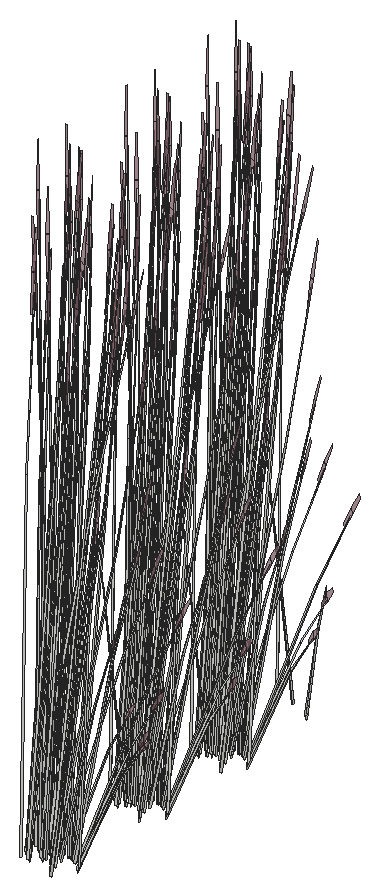
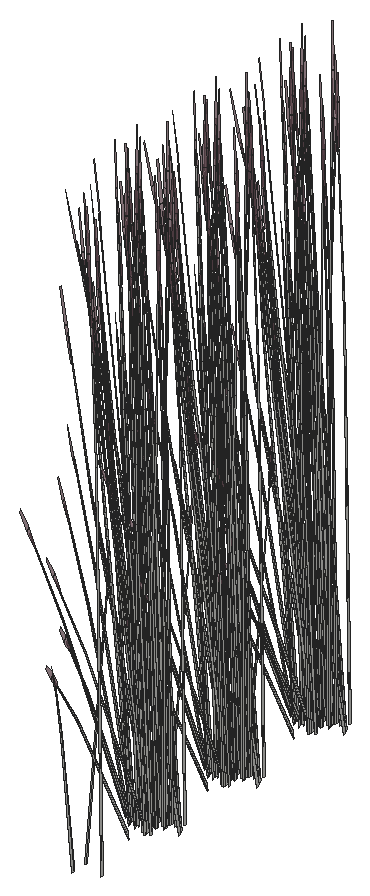
# SketchUp Ruby script. Lengths in inches.
U = 1.inch
M = Sketchup.active_model
def pt(a) = Geom::Point3d.new(a.map { |v| v * U })
def face(e, loops, mat)
  f = e.add_face(loops[0].map { |a| pt(a) })
  loops[1..].each { |l| e.add_face(l.map { |a| pt(a) }).erase! }
  f.material = f.back_material = mat if mat
  f
end
# faces: each face lists its corners as indices into pts; further lists are holes
def faces(e, pts, list, mat = nil) = list.each { |f| face(e, (f[0].is_a?(Array) ? f : [f]).map { |l| l.map { |i| pts[i] } }, mat) }
# xy, xz, yz: faces in a plane at the given z, y or x. An outline is a flat list of corners, or four numbers for a rectangle; further outlines are holes
def ring(l) = l.size == 4 ? [[l[0], l[1]], [l[2], l[1]], [l[2], l[3]], [l[0], l[3]]] : l.each_slice(2).to_a
def flat(e, list, mat, &to3) = list.each { |f| face(e, (f[0].is_a?(Array) ? f : [f]).map { |l| ring(l).map { |u, v| to3.(u, v) } }, mat) }
def xy(e, z, list, mat = nil) = flat(e, list, mat) { |x, y| [x, y, z] }
def xz(e, y, list, mat = nil) = flat(e, list, mat) { |x, z| [x, y, z] }
def yz(e, x, list, mat = nil) = flat(e, list, mat) { |y, z| [x, y, z] }
def lines(e, pts, list) = list.each { |a, b| e.add_line(pt(pts[a]), pt(pts[b])) }
# prism: a flat outline (further loops are holes) pulled along v
def prism(e, loops, v, mat = nil)
  f = face(e, loops, mat); d = Geom::Vector3d.new(v.map { |x| x * U })
  f.pushpull(f.normal.samedirection?(d) ? d.length : -d.length)
end
def box(e, o, s, mat = nil) = prism(e, [[o, [o[0] + s[0], o[1], o[2]], [o[0] + s[0], o[1] + s[1], o[2]], [o[0], o[1] + s[1], o[2]]]], [0, 0, s[2]], mat)
def at(x, y, z, deg = 0) = Geom::Transformation.translation(pt([x, y, z])) * Geom::Transformation.rotation(ORIGIN, Z_AXIS, deg.degrees)
def axes(o, x, y, z) = Geom::Transformation.new([*x, 0, *y, 0, *z, 0, *pt(o).to_a, 1])
def part(name) = M.definitions.add(name)
# library, detail: a bought-in or finely detailed component or shape, given as its bounding box
def library(name, o, s) = part(name).tap { |d| box(d.entities, o, s) }
def detail(e, o, s) = box(e.add_group.entities, o, s)
def put(e, d, t, mat = nil) = e.add_instance(d, t).tap { |i| i.material = mat if mat }
def group(e, t, mat = nil) = e.add_group.tap { |g| g.transformation = t; g.material = mat if mat }.entities
root = M.entities
M.materials.add("LightPink_Translucent").color = [144, 107, 117]
M.materials["LightPink_Translucent"].alpha = 0.75
c1 = part("blade")
p = [[2.15,0.21,22],[0,0.17,0],[0.09,0.45,0],[2.18,0.31,22],[2.29,0.31,22],[0.38,0.45,0],
  [2.48,0.24,33],[2.49,0.24,33],[2.48,0.22,33]]
faces(c1.entities,p,[[0,1,2,3],[4,5,2,3],[6,3,4,7],[8,0,3,6]])
c2 = part("seeds")
p = [[0.3,-0.1,1.38],[-0.01,-0.03,1.59],[-0.01,-0.03,0.03],[0.14,-0.07,-0.07],[0.29,-0.03,3],[0.15,0.01,3.11]]
faces(c2.entities,p,[[0,1,2,3],[1,0,4,5]],"LightPink_Translucent")
c3 = part("blade with seeds")
put(c3.entities,c1,at(0,0,0))
put(c3.entities,c2,axes([2.4,0.25,30.99],[1.5799,-0.05474,1.17369],[-0.12525,1.92788,0.29478],[-0.07173,-0.02425,1.56792]))
put(root,c3,axes([335.77,275.2,49.32],[-0.07557,-0.03078,1.55816],[-0.19412,-0.34391,-0.23804],[0.13095,-0.09333,0.26541]))
put(root,c3,axes([332.92,275.27,50.1],[-0.31568,-0.39156,0],[0.52815,-0.21836,-0.456],[0.12029,-0.04973,1.44655]))
put(root,c3,axes([333.35,275.21,49.78],[0.47255,-0.19538,-0.43871],[0.28245,0.35034,0],[0.10763,-0.0445,1.3917]))
put(root,c3,axes([336.15,275.89,50.29],[-0.18038,-0.01157,1.26356],[-0.18479,-0.31048,-0.27174],[0.22159,-0.08783,0.54024]))
put(root,c3,axes([333.91,276.01,49.82],[0.34009,-0.2937,-0.55095],[0.42248,0.26632,-0.1446],[0.13628,-0.07327,1.21613]))
put(root,c3,axes([333.54,276.35,50.36],[-0.05884,-0.44587,-0.25709],[0.6128,-0.02696,-0.44182],[0.10791,-0.05939,1.41118]))
put(root,c3,axes([333.46,275.37,49.79],[0.47106,0.09668,-0.27372],[-0.11861,0.34048,0.27372],[0.09497,-0.03926,1.22797]))
put(root,c3,axes([333.62,276.7,50.15],[0.56891,0.18939,0.21263],[-0.2738,0.39352,0.44182],[0,-0.09071,1.41855]))
put(root,c3,axes([333.44,276.4375,50.4],[-0.54829,0.02412,0.39531],[-0.04958,-0.40041,-0.19025],[0.09816,-0.04058,1.26923]))
put(root,c3,axes([335.24,275.37,50.1],[0.31568,-0.39156,0],[0.52815,0.21836,-0.456],[0.12029,0.04973,1.44655]))
put(root,c3,axes([336.49,276.92,49.75],[-0.3252,0.04689,1.25103],[-0.05176,-0.37326,0.07161],[0.22777,-0.0565,0.71188]))
put(root,c3,axes([337.08,276.59,50],[-0.31304,-0.24986,-0.05733],[0.34284,-0.22894,-0.25992],[0.09714,-0.01612,0.85731]))
put(root,c3,axes([334.21,276.62,49.95],[0,-0.45213,0],[0.63136,0,0],[0,0,1.58567]))
put(root,c3,axes([334.97,275.57,50.19],[-0.47255,-0.19538,0.43871],[0.28245,-0.35034,0],[0.10763,0.0445,1.3917]))
put(root,c3,axes([333.91,276.33,50.09],[-0.41865,0.35461,0.40429],[-0.49737,-0.31303,0.15865],[0.10093,-0.03539,1.40366]))
put(root,c3,axes([333.18,275.75,50.1875],[-0.14586,0.38834,0.15589],[-0.53375,-0.1099,0.31002],[0.0922,-0.00189,1.41735]))
put(root,c3,axes([332.96,276.0625,49.41],[-0.49699,0.15644,1.13921],[-0.15819,-0.44887,0.44265],[0.30518,0.00747,1.29573]))
put(root,c3,axes([334.29,276.18,50.3125],[0.09741,-0.34873,0.12794],[0.4759,0.06053,-0.36534],[0.08661,0.03581,1.11991]))
put(root,c3,axes([336.84,276.67,49.32],[-0.02639,-0.05932,1.55816],[0.18302,-0.34702,-0.23804],[0.18462,-0.00499,0.26541]))
put(root,c3,axes([334.09,276.27,50.4],[-0.30332,-0.32798,0.39531],[0.45944,-0.23096,-0.19025],[0.09816,0.04058,1.26923]))
put(root,c3,axes([334.25,276.3,50.36],[0.50979,-0.25942,-0.25709],[0.339,0.36656,-0.44182],[0.12578,0.03723,1.41118]))
put(root,c3,axes([335.53,275.61,49.78],[0.47255,0.19538,-0.43871],[-0.28245,0.35034,0],[0.10763,0.0445,1.3917]))
put(root,c3,axes([334.63,276.72,49.95],[0.56491,0,0],[0,0.40454,0],[0,0,1.5764]))
put(root,c3,axes([334.79,275.77,50.1875],[-0.54257,0.10371,0.15589],[-0.13397,-0.38597,0.31002],[0.04839,0.05624,1.41735]))
put(root,c3,axes([335.4,275.75,49.79],[0.11861,0.34048,-0.27372],[-0.47106,0.09668,0.27372],[0.09497,0.03926,1.22797]))
put(root,c3,axes([334.45,276.51,50.1],[-0.63817,-0.08233,0.43472],[0.12987,-0.46497,0.17059],[0.09326,0.0449,1.50931]))
put(root,c3,axes([334.56,277.62,49.93],[0.53009,-0.13258,-0.16963],[0.18627,0.38191,0.00007],[0.05851,-0.01465,1.53656]))
put(root,c3,axes([334.62,276.89,49.96],[0.35245,0.2524,0],[-0.35245,0.2524,0],[0,0,1.49564]))
put(root,c3,axes([335.58,276.78,50.1875],[-0.39671,-0.28463,0.15589],[0.39978,-0.27607,0.31002],[-0.04381,0.05813,1.41735]))
put(root,c3,axes([334.84,276.35,49.82],[0.52523,0.06406,-0.55095],[-0.11084,0.39517,-0.1446],[0.15674,0.04788,1.21613]))
put(root,c3,axes([337.16,277.04,50.44],[-0.31197,0.06451,1.01491],[0.14684,-0.26661,0.74569],[0.1655,0.01824,0.22354]))
put(root,c3,axes([334.62,276.6,50.4],[0.24498,-0.3521,0.39531],[0.50902,0.16945,-0.19025],[0,0.08116,1.26923]))
put(root,c3,axes([334.52,276.8,50.03],[0,0.45191,-0.04981],[-0.63136,0,0],[0,0.0142,1.58489]))
put(root,c3,axes([334.57,276.48,49.95],[0.30332,0.32798,-0.39531],[-0.45944,0.23096,0.19025],[0.09816,0.04058,1.26923]))
put(root,c3,axes([335.9,276.8,50.19],[0,-0.39075,0.43871],[0.56491,0,0],[0,0.089,1.3917]))
put(root,c3,axes([334.83,276.68,50.3125],[0.47043,-0.11396,0.12794],[0.16474,0.32541,-0.36534],[0,0.07162,1.11991]))
put(root,c3,axes([336.58,277.47,50.29],[-0.1216,-0.0961,1.26356],[0.15822,-0.31792,-0.27174],[0.24603,0.04307,0.54024]))
put(root,c3,axes([334.4,277.82,49.95],[0.50902,0.17543,0],[-0.24498,0.36452,0],[0,0,1.54589]))
put(root,c3,axes([334.22,277.67,50.02],[0.21952,0.44891,-0.05313],[-0.62724,0.1573,0],[0.00767,0.01568,1.52132]))
put(root,c3,axes([336.29,276.86,50.1],[0.63136,0,0],[0,0.43672,-0.456],[0,0.09947,1.44655]))
put(root,c3,axes([336.03,277.09,49.94],[-0.63105,-0.00312,-0.04397],[0,-0.43672,0.44129],[-0.01983,0.09942,1.3992]))
put(root,c3,axes([334.67,276.71,50.36],[0.56863,0.18645,-0.25709],[-0.2738,0.39352,-0.44182],[0.01787,0.09662,1.41118]))
put(root,c3,axes([335.9,277.15,49.79],[-0.35245,0.2438,-0.27372],[-0.35245,-0.2438,0.27372],[0,0.07853,1.22797]))
put(root,c3,axes([336.15,277.16,49.78],[0,0.39075,-0.43871],[-0.56491,0,0],[0,0.089,1.3917]))
put(root,c3,axes([335.43,277.97,50.44],[-0.28429,-0.11236,1.01491],[0.36709,-0.11416,0.74569],[0.09901,0.0967,0.22354]))
put(root,c3,axes([335.51,278.39,49.32],[0.03679,-0.05641,1.55816],[0.46313,-0.16615,-0.23804],[0.14041,0.08599,0.26541]))
put(root,c3,axes([334.9,277.1,49.85],[0.18514,0.35777,-0.61156],[-0.53331,0.12885,-0.16051],[0.02046,0.12115,1.3499]))
put(root,c3,axes([335.47,278.48,50.36],[-0.32378,-0.01225,0.92831],[0.21383,-0.26028,0.51254],[0.12791,0.09247,0.72818]))
put(root,c3,axes([334.42,277.85,50.29],[0.00891,-0.12953,1.26356],[0.4258,-0.14469,-0.27174],[0.13144,0.15503,0.54024]))
put(root,c3,axes([334.77,284.76,50.29],[-0.14352,0.07909,1.26356],[-0.42983,-0.13843,-0.27174],[0.07968,-0.17216,0.54024]))
put(root,c3,axes([335.77,285,49.32],[-0.07557,-0.03078,1.55816],[-0.19412,-0.34391,-0.23804],[0.13095,-0.09333,0.26541]))
put(root,c3,axes([332.92,285.07,50.1],[-0.31568,-0.39156,0],[0.52815,-0.21836,-0.456],[0.12029,-0.04973,1.44655]))
put(root,c3,axes([333.35,285.01,49.78],[0.47255,-0.19538,-0.43871],[0.28245,0.35034,0],[0.10763,-0.0445,1.3917]))
put(root,c3,axes([336.15,285.6875,50.29],[-0.18038,-0.01157,1.26356],[-0.18479,-0.31048,-0.27174],[0.22159,-0.08783,0.54024]))
put(root,c3,axes([333.91,285.81,49.82],[0.34009,-0.2937,-0.55095],[0.42248,0.26632,-0.1446],[0.13628,-0.07327,1.21613]))
put(root,c3,axes([333.54,286.15,50.36],[-0.05884,-0.44587,-0.25709],[0.6128,-0.02696,-0.44182],[0.10791,-0.05939,1.41118]))
put(root,c3,axes([333.46,285.17,49.79],[0.47106,0.09668,-0.27372],[-0.11861,0.34048,0.27372],[0.09497,-0.03926,1.22797]))
put(root,c3,axes([333.62,286.5,50.15],[0.56891,0.18939,0.21263],[-0.2738,0.39352,0.44182],[0,-0.09071,1.41855]))
put(root,c3,axes([333.44,286.24,50.4],[-0.54829,0.02412,0.39531],[-0.04958,-0.40041,-0.19025],[0.09816,-0.04058,1.26923]))
put(root,c3,axes([335.24,285.17,50.1],[0.31568,-0.39156,0],[0.52815,0.21836,-0.456],[0.12029,0.04973,1.44655]))
put(root,c3,axes([336.49,286.72,49.75],[-0.3252,0.04689,1.25103],[-0.05176,-0.37326,0.07161],[0.22777,-0.0565,0.71188]))
put(root,c3,axes([337.08,286.39,50],[-0.31304,-0.24986,-0.05733],[0.34284,-0.22894,-0.25992],[0.09714,-0.01612,0.85731]))
put(root,c3,axes([334.21,286.42,49.95],[0,-0.45213,0],[0.63136,0,0],[0,0,1.58567]))
put(root,c3,axes([334.97,285.375,50.19],[-0.47255,-0.19538,0.43871],[0.28245,-0.35034,0],[0.10763,0.0445,1.3917]))
put(root,c3,axes([333.91,286.14,50.09],[-0.41865,0.35461,0.40429],[-0.49737,-0.31303,0.15865],[0.10093,-0.03539,1.40366]))
put(root,c3,axes([333.18,285.55,50.1875],[-0.14586,0.38834,0.15589],[-0.53375,-0.1099,0.31002],[0.0922,-0.00189,1.41735]))
put(root,c3,axes([332.96,285.87,49.41],[-0.49699,0.15644,1.13921],[-0.15819,-0.44887,0.44265],[0.30518,0.00747,1.29573]))
put(root,c3,axes([334.29,285.98,50.3125],[0.09741,-0.34873,0.12794],[0.4759,0.06053,-0.36534],[0.08661,0.03581,1.11991]))
put(root,c3,axes([336.84,286.48,49.32],[-0.02639,-0.05932,1.55816],[0.18302,-0.34702,-0.23804],[0.18462,-0.00499,0.26541]))
put(root,c3,axes([334.09,286.08,50.4],[-0.30332,-0.32798,0.39531],[0.45944,-0.23096,-0.19025],[0.09816,0.04058,1.26923]))
put(root,c3,axes([334.25,286.1,50.36],[0.50979,-0.25942,-0.25709],[0.339,0.36656,-0.44182],[0.12578,0.03723,1.41118]))
put(root,c3,axes([335.53,285.41,49.78],[0.47255,0.19538,-0.43871],[-0.28245,0.35034,0],[0.10763,0.0445,1.3917]))
put(root,c3,axes([334.63,286.52,49.95],[0.56491,0,0],[0,0.40454,0],[0,0,1.5764]))
put(root,c3,axes([334.79,285.57,50.1875],[-0.54257,0.10371,0.15589],[-0.13397,-0.38597,0.31002],[0.04839,0.05624,1.41735]))
put(root,c3,axes([335.4,285.55,49.79],[0.11861,0.34048,-0.27372],[-0.47106,0.09668,0.27372],[0.09497,0.03926,1.22797]))
put(root,c3,axes([334.45,286.32,50.1],[-0.63817,-0.08233,0.43472],[0.12987,-0.46497,0.17059],[0.09326,0.0449,1.50931]))
put(root,c3,axes([334.56,287.42,49.93],[0.53009,-0.13258,-0.16963],[0.18627,0.38191,0.00007],[0.05851,-0.01465,1.53656]))
put(root,c3,axes([334.62,286.7,49.96],[0.35245,0.2524,0],[-0.35245,0.2524,0],[0,0,1.49564]))
put(root,c3,axes([335.58,286.59,50.1875],[-0.39671,-0.28463,0.15589],[0.39978,-0.27607,0.31002],[-0.04381,0.05813,1.41735]))
put(root,c3,axes([334.84,286.16,49.82],[0.52523,0.06406,-0.55095],[-0.11084,0.39517,-0.1446],[0.15674,0.04788,1.21613]))
put(root,c3,axes([334.62,286.4,50.4],[0.24498,-0.3521,0.39531],[0.50902,0.16945,-0.19025],[0,0.08116,1.26923]))
put(root,c3,axes([334.52,286.6,50.03],[0,0.45191,-0.04981],[-0.63136,0,0],[0,0.0142,1.58489]))
put(root,c3,axes([334.57,286.28,49.95],[0.30332,0.32798,-0.39531],[-0.45944,0.23096,0.19025],[0.09816,0.04058,1.26923]))
put(root,c3,axes([335.9,286.6,50.19],[0,-0.39075,0.43871],[0.56491,0,0],[0,0.089,1.3917]))
put(root,c3,axes([334.83,286.48,50.3125],[0.47043,-0.11396,0.12794],[0.16474,0.32541,-0.36534],[0,0.07162,1.11991]))
put(root,c3,axes([336.58,287.27,50.29],[-0.1216,-0.0961,1.26356],[0.15822,-0.31792,-0.27174],[0.24603,0.04307,0.54024]))
put(root,c3,axes([334.4,287.625,49.95],[0.50902,0.17543,0],[-0.24498,0.36452,0],[0,0,1.54589]))
put(root,c3,axes([334.22,287.48,50.02],[0.21952,0.44891,-0.05313],[-0.62724,0.1573,0],[0.00767,0.01568,1.52132]))
put(root,c3,axes([336.29,286.66,50.1],[0.63136,0,0],[0,0.43672,-0.456],[0,0.09947,1.44655]))
put(root,c3,axes([336.03,286.89,49.94],[-0.63105,-0.00312,-0.04397],[0,-0.43672,0.44129],[-0.01983,0.09942,1.3992]))
put(root,c3,axes([334.67,286.51,50.36],[0.56863,0.18645,-0.25709],[-0.2738,0.39352,-0.44182],[0.01787,0.09662,1.41118]))
put(root,c3,axes([335.9,286.95,49.79],[-0.35245,0.2438,-0.27372],[-0.35245,-0.2438,0.27372],[0,0.07853,1.22797]))
put(root,c3,axes([336.15,286.96,49.78],[0,0.39075,-0.43871],[-0.56491,0,0],[0,0.089,1.3917]))
put(root,c3,axes([335.51,288.1875,49.32],[0.03679,-0.05641,1.55816],[0.46313,-0.16615,-0.23804],[0.14041,0.08599,0.26541]))
put(root,c3,axes([334.9,286.91,49.85],[0.18514,0.35777,-0.61156],[-0.53331,0.12885,-0.16051],[0.02046,0.12115,1.3499]))
put(root,c3,axes([335.47,288.28,50.36],[-0.32378,-0.01225,0.92831],[0.21383,-0.26028,0.51254],[0.12791,0.09247,0.72818]))
put(root,c3,axes([334.42,287.65,50.29],[0.00891,-0.12953,1.26356],[0.4258,-0.14469,-0.27174],[0.13144,0.15503,0.54024]))
put(root,c3,axes([334.77,293.73,50.29],[-0.14352,0.07909,1.26356],[-0.42983,-0.13843,-0.27174],[0.07968,-0.17216,0.54024]))
put(root,c3,axes([335.77,293.98,49.32],[-0.07557,-0.03078,1.55816],[-0.19412,-0.34391,-0.23804],[0.13095,-0.09333,0.26541]))
put(root,c3,axes([332.92,294.05,50.1],[-0.31568,-0.39156,0],[0.52815,-0.21836,-0.456],[0.12029,-0.04973,1.44655]))
put(root,c3,axes([333.35,293.99,49.78],[0.47255,-0.19538,-0.43871],[0.28245,0.35034,0],[0.10763,-0.0445,1.3917]))
put(root,c3,axes([336.15,294.67,50.29],[-0.18038,-0.01157,1.26356],[-0.18479,-0.31048,-0.27174],[0.22159,-0.08783,0.54024]))
put(root,c3,axes([333.91,294.79,49.82],[0.34009,-0.2937,-0.55095],[0.42248,0.26632,-0.1446],[0.13628,-0.07327,1.21613]))
put(root,c3,axes([333.54,295.13,50.36],[-0.05884,-0.44587,-0.25709],[0.6128,-0.02696,-0.44182],[0.10791,-0.05939,1.41118]))
put(root,c3,axes([333.46,294.14,49.79],[0.47106,0.09668,-0.27372],[-0.11861,0.34048,0.27372],[0.09497,-0.03926,1.22797]))
put(root,c3,axes([333.62,295.48,50.15],[0.56891,0.18939,0.21263],[-0.2738,0.39352,0.44182],[0,-0.09071,1.41855]))
put(root,c3,axes([333.44,295.22,50.4],[-0.54829,0.02412,0.39531],[-0.04958,-0.40041,-0.19025],[0.09816,-0.04058,1.26923]))
put(root,c3,axes([335.24,294.15,50.1],[0.31568,-0.39156,0],[0.52815,0.21836,-0.456],[0.12029,0.04973,1.44655]))
put(root,c3,axes([336.49,295.7,49.75],[-0.3252,0.04689,1.25103],[-0.05176,-0.37326,0.07161],[0.22777,-0.0565,0.71188]))
put(root,c3,axes([337.08,295.37,50],[-0.31304,-0.24986,-0.05733],[0.34284,-0.22894,-0.25992],[0.09714,-0.01612,0.85731]))
put(root,c3,axes([334.21,295.4,49.95],[0,-0.45213,0],[0.63136,0,0],[0,0,1.58567]))
put(root,c3,axes([334.97,294.35,50.19],[-0.47255,-0.19538,0.43871],[0.28245,-0.35034,0],[0.10763,0.0445,1.3917]))
put(root,c3,axes([333.91,295.11,50.09],[-0.41865,0.35461,0.40429],[-0.49737,-0.31303,0.15865],[0.10093,-0.03539,1.40366]))
put(root,c3,axes([333.18,294.53,50.1875],[-0.14586,0.38834,0.15589],[-0.53375,-0.1099,0.31002],[0.0922,-0.00189,1.41735]))
put(root,c3,axes([332.96,294.84,49.41],[-0.49699,0.15644,1.13921],[-0.15819,-0.44887,0.44265],[0.30518,0.00747,1.29573]))
put(root,c3,axes([334.29,294.96,50.3125],[0.09741,-0.34873,0.12794],[0.4759,0.06053,-0.36534],[0.08661,0.03581,1.11991]))
put(root,c3,axes([336.84,295.45,49.32],[-0.02639,-0.05932,1.55816],[0.18302,-0.34702,-0.23804],[0.18462,-0.00499,0.26541]))
put(root,c3,axes([334.09,295.05,50.4],[-0.30332,-0.32798,0.39531],[0.45944,-0.23096,-0.19025],[0.09816,0.04058,1.26923]))
put(root,c3,axes([334.25,295.07,50.36],[0.50979,-0.25942,-0.25709],[0.339,0.36656,-0.44182],[0.12578,0.03723,1.41118]))
put(root,c3,axes([335.53,294.39,49.78],[0.47255,0.19538,-0.43871],[-0.28245,0.35034,0],[0.10763,0.0445,1.3917]))
put(root,c3,axes([334.63,295.5,49.95],[0.56491,0,0],[0,0.40454,0],[0,0,1.5764]))
put(root,c3,axes([334.79,294.55,50.1875],[-0.54257,0.10371,0.15589],[-0.13397,-0.38597,0.31002],[0.04839,0.05624,1.41735]))
put(root,c3,axes([335.4,294.53,49.79],[0.11861,0.34048,-0.27372],[-0.47106,0.09668,0.27372],[0.09497,0.03926,1.22797]))
put(root,c3,axes([334.45,295.29,50.1],[-0.63817,-0.08233,0.43472],[0.12987,-0.46497,0.17059],[0.09326,0.0449,1.50931]))
put(root,c3,axes([334.56,296.39,49.93],[0.53009,-0.13258,-0.16963],[0.18627,0.38191,0.00007],[0.05851,-0.01465,1.53656]))
put(root,c3,axes([334.62,295.67,49.96],[0.35245,0.2524,0],[-0.35245,0.2524,0],[0,0,1.49564]))
put(root,c3,axes([335.58,295.5625,50.1875],[-0.39671,-0.28463,0.15589],[0.39978,-0.27607,0.31002],[-0.04381,0.05813,1.41735]))
put(root,c3,axes([334.84,295.13,49.82],[0.52523,0.06406,-0.55095],[-0.11084,0.39517,-0.1446],[0.15674,0.04788,1.21613]))
put(root,c3,axes([334.62,295.38,50.4],[0.24498,-0.3521,0.39531],[0.50902,0.16945,-0.19025],[0,0.08116,1.26923]))
put(root,c3,axes([334.52,295.58,50.03],[0,0.45191,-0.04981],[-0.63136,0,0],[0,0.0142,1.58489]))
put(root,c3,axes([334.57,295.26,49.95],[0.30332,0.32798,-0.39531],[-0.45944,0.23096,0.19025],[0.09816,0.04058,1.26923]))
put(root,c3,axes([335.9,295.57,50.19],[0,-0.39075,0.43871],[0.56491,0,0],[0,0.089,1.3917]))
put(root,c3,axes([334.83,295.46,50.3125],[0.47043,-0.11396,0.12794],[0.16474,0.32541,-0.36534],[0,0.07162,1.11991]))
put(root,c3,axes([336.58,296.25,50.29],[-0.1216,-0.0961,1.26356],[0.15822,-0.31792,-0.27174],[0.24603,0.04307,0.54024]))
put(root,c3,axes([334.4,296.6,49.95],[0.50902,0.17543,0],[-0.24498,0.36452,0],[0,0,1.54589]))
put(root,c3,axes([334.22,296.45,50.02],[0.21952,0.44891,-0.05313],[-0.62724,0.1573,0],[0.00767,0.01568,1.52132]))
put(root,c3,axes([336.29,295.64,50.1],[0.63136,0,0],[0,0.43672,-0.456],[0,0.09947,1.44655]))
put(root,c3,axes([336.03,295.86,49.94],[-0.63105,-0.00312,-0.04397],[0,-0.43672,0.44129],[-0.01983,0.09942,1.3992]))
put(root,c3,axes([334.67,295.48,50.36],[0.56863,0.18645,-0.25709],[-0.2738,0.39352,-0.44182],[0.01787,0.09662,1.41118]))
put(root,c3,axes([335.9,295.93,49.79],[-0.35245,0.2438,-0.27372],[-0.35245,-0.2438,0.27372],[0,0.07853,1.22797]))
put(root,c3,axes([336.15,295.9375,49.78],[0,0.39075,-0.43871],[-0.56491,0,0],[0,0.089,1.3917]))
put(root,c3,axes([335.51,297.16,49.32],[0.03679,-0.05641,1.55816],[0.46313,-0.16615,-0.23804],[0.14041,0.08599,0.26541]))
put(root,c3,axes([334.9,295.88,49.85],[0.18514,0.35777,-0.61156],[-0.53331,0.12885,-0.16051],[0.02046,0.12115,1.3499]))
put(root,c3,axes([335.47,297.26,50.36],[-0.32378,-0.01225,0.92831],[0.21383,-0.26028,0.51254],[0.12791,0.09247,0.72818]))
put(root,c3,axes([334.42,296.63,50.29],[0.00891,-0.12953,1.26356],[0.4258,-0.14469,-0.27174],[0.13144,0.15503,0.54024]))
put(root,c3,axes([334.77,303.22,50.29],[-0.14352,0.07909,1.26356],[-0.42983,-0.13843,-0.27174],[0.07968,-0.17216,0.54024]))
put(root,c3,axes([335.77,303.46,49.32],[-0.07557,-0.03078,1.55816],[-0.19412,-0.34391,-0.23804],[0.13095,-0.09333,0.26541]))
put(root,c3,axes([332.92,303.54,50.1],[-0.31568,-0.39156,0],[0.52815,-0.21836,-0.456],[0.12029,-0.04973,1.44655]))
